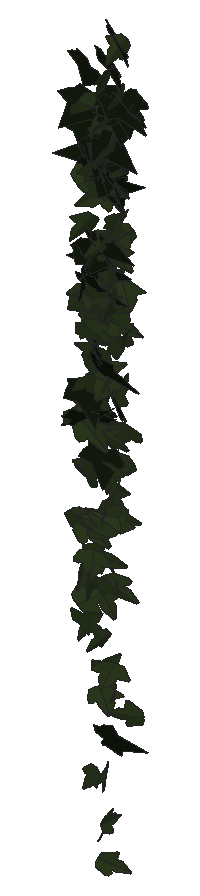
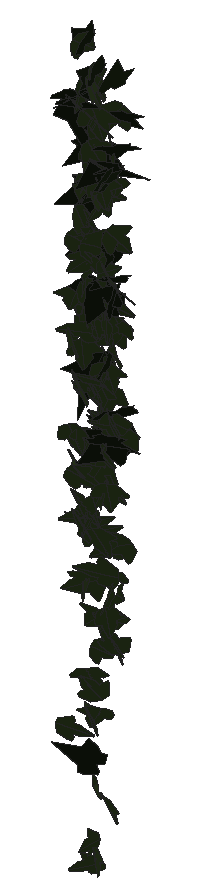
# SketchUp Ruby script. Lengths in inches.
U = 1.inch
M = Sketchup.active_model
def pt(a) = Geom::Point3d.new(a.map { |v| v * U })
def face(e, loops, mat)
  f = e.add_face(loops[0].map { |a| pt(a) })
  loops[1..].each { |l| e.add_face(l.map { |a| pt(a) }).erase! }
  f.material = f.back_material = mat if mat
  f
end
# faces: each face lists its corners as indices into pts; further lists are holes
def faces(e, pts, list, mat = nil) = list.each { |f| face(e, (f[0].is_a?(Array) ? f : [f]).map { |l| l.map { |i| pts[i] } }, mat) }
# xy, xz, yz: faces in a plane at the given z, y or x. An outline is a flat list of corners, or four numbers for a rectangle; further outlines are holes
def ring(l) = l.size == 4 ? [[l[0], l[1]], [l[2], l[1]], [l[2], l[3]], [l[0], l[3]]] : l.each_slice(2).to_a
def flat(e, list, mat, &to3) = list.each { |f| face(e, (f[0].is_a?(Array) ? f : [f]).map { |l| ring(l).map { |u, v| to3.(u, v) } }, mat) }
def xy(e, z, list, mat = nil) = flat(e, list, mat) { |x, y| [x, y, z] }
def xz(e, y, list, mat = nil) = flat(e, list, mat) { |x, z| [x, y, z] }
def yz(e, x, list, mat = nil) = flat(e, list, mat) { |y, z| [x, y, z] }
def lines(e, pts, list) = list.each { |a, b| e.add_line(pt(pts[a]), pt(pts[b])) }
# prism: a flat outline (further loops are holes) pulled along v
def prism(e, loops, v, mat = nil)
  f = face(e, loops, mat); d = Geom::Vector3d.new(v.map { |x| x * U })
  f.pushpull(f.normal.samedirection?(d) ? d.length : -d.length)
end
def box(e, o, s, mat = nil) = prism(e, [[o, [o[0] + s[0], o[1], o[2]], [o[0] + s[0], o[1] + s[1], o[2]], [o[0], o[1] + s[1], o[2]]]], [0, 0, s[2]], mat)
def at(x, y, z, deg = 0) = Geom::Transformation.translation(pt([x, y, z])) * Geom::Transformation.rotation(ORIGIN, Z_AXIS, deg.degrees)
def axes(o, x, y, z) = Geom::Transformation.new([*x, 0, *y, 0, *z, 0, *pt(o).to_a, 1])
def part(name) = M.definitions.add(name)
# library, detail: a bought-in or finely detailed component or shape, given as its bounding box
def library(name, o, s) = part(name).tap { |d| box(d.entities, o, s) }
def detail(e, o, s) = box(e.add_group.entities, o, s)
def put(e, d, t, mat = nil) = e.add_instance(d, t).tap { |i| i.material = mat if mat }
def group(e, t, mat = nil) = e.add_group.tap { |g| g.transformation = t; g.material = mat if mat }.entities
root = M.entities
M.materials.add("1026 AP 7946 SUNNY SIDE UP").color = [254, 231, 186]
M.materials.add("efeu1").color = [18, 25, 13]
M.materials.add("efeu2").color = [43, 57, 29]
c1 = part("ivyleaf_9")
p = [[1.54,2.16,1.25],[1.36,2.04,1.19],[-0.21,0.99,0.68],[-0.71,1.11,0.82],[-0.85,0.86,0.67],[-0.8,0.17,0.21],
  [-0.9,-0.01,0.1],[-0.67,-0.16,-0.02],[-0.08,-0.08,-0.05],[-0.03,-0.6,-0.4],[0.65,-0.88,-0.66],[0.83,-0.6,-0.49],
  [1.29,-0.42,-0.43],[1.8125,-0.07,-0.26],[1.21,0.44,0.15]]
faces(c1.entities,p,[[0,1,2,3,4,5,6,7,8,9,10,11,12,13,14]],"efeu1")
c2 = part("ivyleaf_10")
p = [[0,0.5,-0.03],[-0.0625,2.02,-0.43],[-0.19,2.01,-0.46],[-0.54,1.05,-0.29],[-0.52,0.625,-0.18],[-0.83,0.76,-0.28],
  [-1.16,0.64,-0.33],[-1.15,0.33,-0.24],[-0.77,-0.39,0.02],[-0.3,-0.51,0.16],[0.04,-0.48,0.23],[-0.02,2.01,-0.4375],
  [-0.06,2.01,-0.43],[0.04,-0.49,0.23],[0.67,-0.49,0.14],[1.38,0.36,-0.2],[1.375,0.51,-0.24],[0.81,0.65,-0.19],
  [0.62,0.59,-0.15],[0.6,1.09,-0.28],[0.5,1.23,-0.31]]
faces(c2.entities,p,[[0,1,2,3,4,5,6,7,8,9,10],[11,12,0,13,14,15,16,17,18,19,20]],"efeu2")
put(root,c1,axes([107.27,212.65,259.01],[-0.35146,-0.07913,0.09718],[-0.12704,-0.05448,-0.24347],[0.1468,-0.23659,0.02195]),"1026 AP 7946 SUNNY SIDE UP")
put(root,c1,axes([107.18,212.35,266.29],[-0.33681,-0.14799,0.05374],[-0.04557,-0.05088,-0.26728],[0.24294,-0.21471,0.02438]),"1026 AP 7946 SUNNY SIDE UP")
put(root,c1,axes([107.03,212.51,265.68],[-0.19517,-0.2139,-0.02355],[0.05901,0.00306,-0.25277],[0.33286,-0.12596,0.031]),"1026 AP 7946 SUNNY SIDE UP")
put(root,c2,axes([107.17,212.33,263.53],[-0.07974,-0.19065,0.17247],[-0.03607,-0.16768,-0.20355],[0.39844,-0.05333,0.01609]),"1026 AP 7946 SUNNY SIDE UP")
put(root,c2,axes([107.17,212.68,262.86],[-0.03382,0.04301,-0.23821],[-0.13272,-0.2184,-0.03501],[-0.34559,0.07966,0.03676]),"1026 AP 7946 SUNNY SIDE UP")
put(root,c2,axes([106.9,212.28,256.57],[-0.2205,0.00735,-0.19781],[0.29524,-0.04555,-0.14329],[-0.06456,-0.2334,0.02032]),"1026 AP 7946 SUNNY SIDE UP")
put(root,c2,axes([107.09,212.28,255.36],[0.01346,0.14801,-0.16409],[-0.02486,-0.1594,-0.1536],[-0.34197,0.01742,0.00471]),"1026 AP 7946 SUNNY SIDE UP")
put(root,c1,axes([107.03,212.5,262.22],[-0.00857,-0.00687,-0.25296],[0.26934,-0.17609,0.00013],[-0.27675,-0.17116,0.00796]),"1026 AP 7946 SUNNY SIDE UP")
put(root,c1,axes([107.41,212.5,265.09],[-0.31889,-0.00412,0.17125],[-0.25545,-0.05117,-0.20576],[0.05592,-0.2572,0.03663]),"1026 AP 7946 SUNNY SIDE UP")
put(root,c2,axes([106.97,212.62,259.47],[0.2066,-0.10808,0.16355],[0.19545,-0.09976,-0.17585],[0.23126,0.18086,0.00251]),"1026 AP 7946 SUNNY SIDE UP")
put(root,c2,axes([107.2,212.46,257.8],[-0.29258,-0.10467,0.03754],[-0.03402,-0.03671,-0.21908],[0.17124,-0.18614,0.02062]),"1026 AP 7946 SUNNY SIDE UP")
put(root,c2,axes([106.98,212.2,259.04],[-0.24658,-0.10244,-0.17997],[0.2466,0.0772,-0.19185],[0.20022,-0.22124,0.01466]),"1026 AP 7946 SUNNY SIDE UP")
put(root,c2,axes([107.17,212.33,261.53],[-0.23648,-0.16806,-0.00341],[0.02047,-0.00849,-0.23185],[0.26349,-0.15018,0.01495]),"1026 AP 7946 SUNNY SIDE UP")
put(root,c2,axes([107.17,212.51,255],[-0.13843,-0.20505,0.00708],[0.01022,-0.01152,-0.2297],[0.32251,-0.08765,0.01032]),"1026 AP 7946 SUNNY SIDE UP")
put(root,c2,axes([107.37,212.35,261.97],[-0.14813,-0.02247,0.22162],[-0.25618,-0.14717,-0.09015],[0.22401,-0.18317,0.04346]),"1026 AP 7946 SUNNY SIDE UP")
put(root,c1,axes([107.42,212.48,262.67],[-0.26739,0.15562,0.09575],[-0.13906,0.03865,-0.23536],[-0.24798,-0.18947,0.02874]),"1026 AP 7946 SUNNY SIDE UP")
put(root,c2,axes([107.02,212.32,261.58],[-0.28592,-0.06176,-0.12207],[0.20805,-0.0592,-0.17826],[0.02561,-0.20861,0.0853]),"1026 AP 7946 SUNNY SIDE UP")
put(root,c2,axes([107.4,212.18,257.7],[-0.02531,0.0288,0.2378],[-0.34752,0.06974,-0.02445],[-0.11325,-0.22045,0.02189]),"1026 AP 7946 SUNNY SIDE UP")
put(root,c2,axes([106.95,212.48,260.95],[0.12561,-0.03553,0.21534],[0.27654,-0.11404,-0.08979],[0.18677,0.19275,-0.01187]),"1026 AP 7946 SUNNY SIDE UP")
put(root,c1,axes([106.93,212.15,258.87],[0.24358,0.16582,-0.08438],[0.04295,0.08636,0.23121],[0.28828,-0.15297,0.03684]),"1026 AP 7946 SUNNY SIDE UP")
put(root,c2,axes([107.1875,212.48,261.71],[0.01596,-0.22356,-0.06441],[0.01796,0.06172,-0.22976],[0.36404,0.00675,0.01416]),"1026 AP 7946 SUNNY SIDE UP")
put(root,c2,axes([107.29,212.41,260.49],[-0.31761,-0.05874,0.07705],[-0.09814,-0.05161,-0.21476],[0.11338,-0.20924,0.02994]),"1026 AP 7946 SUNNY SIDE UP")
put(root,c1,axes([107.07,212.375,259.57],[-0.0634,-0.24999,-0.08098],[0.0215,0.07598,-0.26042],[0.41083,-0.04255,0.00113]),"1026 AP 7946 SUNNY SIDE UP")
put(root,c1,axes([107,212.5625,262.72],[0.03438,-0.21108,-0.12315],[0.07119,0.12029,-0.21172],[0.37379,-0.00349,0.05165]),"1026 AP 7946 SUNNY SIDE UP")
put(root,c2,axes([107.26,212.52,261.58],[-0.15796,-0.16653,0.15001],[-0.02283,-0.1556,-0.19331],[0.34807,-0.08578,0.0554]),"1026 AP 7946 SUNNY SIDE UP")
put(root,c2,axes([107.41,212.47,258.61],[0.02727,-0.04688,-0.22961],[-0.25417,0.15457,-0.0456],[0.25172,0.16115,-0.02117]),"1026 AP 7946 SUNNY SIDE UP")
put(root,c2,axes([107.2,212.24,254.21],[0.23113,-0.16519,0.00378],[-0.0126,-0.01329,-0.22737],[0.25955,0.14646,-0.01441]),"1026 AP 7946 SUNNY SIDE UP")
put(root,c2,axes([106.93,212.38,259.3],[0.17451,0.00598,-0.2306],[0.34215,0.05624,0.113],[0.08332,-0.24346,0.01894]),"1026 AP 7946 SUNNY SIDE UP")
put(root,c1,axes([107.11,212.43,267.02],[-0.12747,-0.16973,0.22097],[0.05951,-0.22944,-0.17288],[0.42715,-0.01868,0.09002]),"1026 AP 7946 SUNNY SIDE UP")
put(root,c2,axes([107.28,212.6,264.8],[-0.17533,-0.21789,0.03418],[-0.00679,-0.0364,-0.25203],[0.3468,-0.11087,0.01234]),"1026 AP 7946 SUNNY SIDE UP")
put(root,c2,axes([107.27,212.37,250.64],[0.24317,-0.14595,-0.03879],[-0.05607,0.01578,-0.21858],[0.22995,0.15819,-0.01227]),"1026 AP 7946 SUNNY SIDE UP")
put(root,c2,axes([107.11,212.26,254.15],[-0.27249,-0.04333,0.12948],[0.18418,0.04877,0.18362],[-0.09967,0.2086,-0.01469]),"1026 AP 7946 SUNNY SIDE UP")
put(root,c2,axes([107.24,212.48,262.9375],[0.17205,-0.24274,0.06822],[0.01884,-0.0686,-0.27416],[0.39576,0.1088,-0.01661]),"1026 AP 7946 SUNNY SIDE UP")
put(root,c1,axes([107.07,212.375,258.85],[0.34957,0.09701,0.06558],[0.10388,0.00581,-0.24896],[-0.1494,0.23102,-0.01968]),"1026 AP 7946 SUNNY SIDE UP")
put(root,c2,axes([107.15,212.17,266.31],[-0.16406,-0.14583,-0.22076],[0.22089,0.16126,-0.18328],[0.34124,-0.1745,0.01251]),"1026 AP 7946 SUNNY SIDE UP")
put(root,c1,axes([107.12,212.71,264.95],[0.05226,-0.20326,0.1472],[0.0136,-0.14429,-0.21265],[0.39148,0.03215,-0.01226]),"1026 AP 7946 SUNNY SIDE UP")
put(root,c2,axes([107.25,212.27,259.89],[-0.1655,-0.20571,-0.12208],[0.11652,0.09334,-0.23653],[0.35368,-0.12701,0.0208]),"1026 AP 7946 SUNNY SIDE UP")
put(root,c2,axes([107.36,212.16,260.39],[-0.01595,0.04964,0.25947],[-0.15963,0.23043,-0.04971],[-0.37027,-0.10148,0.01025]),"1026 AP 7946 SUNNY SIDE UP")
put(root,c1,axes([107.16,212.6,264.88],[-0.07846,-0.17988,0.17531],[0.06463,-0.17819,-0.18158],[0.38508,-0.00674,0.0662]),"1026 AP 7946 SUNNY SIDE UP")
put(root,c2,axes([107.12,212.2,254.6875],[0.18937,0.03532,-0.19977],[0.23407,0.133,0.12085],[0.20362,-0.18574,0.04686]),"1026 AP 7946 SUNNY SIDE UP")
put(root,c2,axes([107.04,212.55,259.37],[0.13889,0.00108,0.21341],[0.32564,-0.00545,-0.09098],[0.00722,0.22513,-0.00191]),"1026 AP 7946 SUNNY SIDE UP")
put(root,c2,axes([107.18,212.33,265.4],[-0.02226,0.04386,-0.26264],[0.11906,-0.2437,-0.04891],[-0.38936,-0.07703,0.00006]),"1026 AP 7946 SUNNY SIDE UP")
put(root,c1,axes([107.28,212.33,265.1875],[-0.01754,0.02952,-0.30196],[-0.14028,0.27939,0.0341],[0.44175,0.08989,-0.00116]),"1026 AP 7946 SUNNY SIDE UP")
put(root,c2,axes([107.33,212.64,264.6],[0.06378,-0.2093,0.11974],[0.01986,-0.11706,-0.22014],[0.37684,0.0416,-0.00866]),"1026 AP 7946 SUNNY SIDE UP")
put(root,c2,axes([107.37,212.11,255.22],[0.04121,-0.10601,-0.2445],[0.02175,0.23817,-0.1069],[0.40727,-0.002,0.03045]),"1026 AP 7946 SUNNY SIDE UP")
put(root,c2,axes([107.45,212.55,266.27],[-0.32454,-0.1257,0.07048],[-0.0637,-0.06513,-0.24698],[0.2164,-0.20769,0.03301]),"1026 AP 7946 SUNNY SIDE UP")
put(root,c2,axes([107.49,212.44,262.03],[-0.28562,0.08917,0.10765],[-0.17145,0.01042,-0.20536],[-0.13038,-0.20904,0.03423]),"1026 AP 7946 SUNNY SIDE UP")
put(root,c2,axes([107.4,212.25,264.9],[-0.07921,-0.25029,0.02683],[-0.00115,-0.02786,-0.26314],[0.39592,-0.05016,0.0046]),"1026 AP 7946 SUNNY SIDE UP")
put(root,c2,axes([107.52,212.44,256.65],[-0.28147,-0.05873,0.11833],[-0.15363,-0.06743,-0.19222],[0.13318,-0.20191,0.02836]),"1026 AP 7946 SUNNY SIDE UP")
put(root,c1,axes([107.15,212.4,263.18],[0.27025,-0.19402,0.00815],[-0.00976,-0.01752,-0.2666],[0.30526,0.17121,-0.01574]),"1026 AP 7946 SUNNY SIDE UP")
put(root,c2,axes([107.19,212.14,264.53],[0.1908,0.06517,-0.23116],[0.23299,0.17456,0.13558],[0.28481,-0.18647,0.04395]),"1026 AP 7946 SUNNY SIDE UP")
put(root,c2,axes([107.43,212.66,265.6],[-0.13892,-0.2061,0.10543],[-0.02164,-0.10594,-0.23002],[0.36201,-0.08543,0.02671]),"1026 AP 7946 SUNNY SIDE UP")
put(root,c2,axes([107.32,212.29,258.89],[-0.10809,0.20697,-0.09447],[0.03483,-0.09046,-0.22509],[-0.355,-0.07189,0.00668]),"1026 AP 7946 SUNNY SIDE UP")
put(root,c2,axes([107.15,212.24,256.38],[0.16936,0.10899,0.18382],[0.2284,0.10441,-0.15596],[-0.23533,0.17978,-0.01907]),"1026 AP 7946 SUNNY SIDE UP")
put(root,c2,axes([107.32,212.4,264.29],[-0.01192,-0.16702,-0.20093],[0.13893,0.18055,-0.16256],[0.37791,-0.07164,0.05342]),"1026 AP 7946 SUNNY SIDE UP")
put(root,c2,axes([107.31,212.24,255.77],[0.34273,0.05747,0.01362],[0.02812,-0.01748,-0.23127],[-0.08825,0.21765,-0.0208]),"1026 AP 7946 SUNNY SIDE UP")
put(root,c1,axes([107.36,212.4375,262.32],[0.29756,0.17356,-0.04665],[-0.03678,-0.04283,-0.2643],[-0.28004,0.19005,-0.01486]),"1026 AP 7946 SUNNY SIDE UP")
put(root,c2,axes([107.36,212.49,257.67],[-0.20351,0.15796,-0.06452],[0.04287,-0.05954,-0.21009],[-0.26425,-0.13131,0.01561]),"1026 AP 7946 SUNNY SIDE UP")
put(root,c1,axes([107.27,212.51,260.51],[0.00841,-0.12603,0.22475],[0.01649,-0.21863,-0.13123],[0.3968,0.01176,0.00069]),"1026 AP 7946 SUNNY SIDE UP")
put(root,c2,axes([107.4,212.45,261.42],[0.1389,-0.19141,0.11355],[-0.05421,0.10649,0.21746],[-0.34391,-0.09409,0.01158]),"1026 AP 7946 SUNNY SIDE UP")
put(root,c2,axes([107.49,212.46,249.43],[0.05444,-0.16766,-0.12683],[-0.05394,0.11752,-0.17548],[0.32169,0.04808,-0.00796]),"1026 AP 7946 SUNNY SIDE UP")
put(root,c2,axes([107.37,212.24,261.87],[0.13209,0.21012,0.07936],[0.03262,0.07333,-0.23256],[-0.34973,0.0862,0.00828]),"1026 AP 7946 SUNNY SIDE UP")
put(root,c2,axes([107.33,212.13,261.21],[-0.2739,-0.05275,-0.13983],[0.2116,0.02136,-0.18675],[0.08637,-0.21961,0.01406]),"1026 AP 7946 SUNNY SIDE UP")
put(root,c1,axes([107.14,212.32,261.98],[0.20909,-0.06903,0.21165],[0.25418,-0.12966,-0.15313],[0.22789,0.20795,-0.0234]),"1026 AP 7946 SUNNY SIDE UP")
put(root,c2,axes([107.53,212.44,259.95],[0.18685,-0.20218,-0.06677],[-0.06711,0.04866,-0.24101],[0.32647,0.12572,-0.01133]),"1026 AP 7946 SUNNY SIDE UP")
put(root,c2,axes([107.61,212.29,264.35],[0.11942,0.0958,-0.25708],[-0.25345,-0.19125,-0.12702],[-0.33631,0.17815,0.00444]),"1026 AP 7946 SUNNY SIDE UP")
put(root,c2,axes([107.5,212.6,266.98],[0.09253,-0.24822,0.06104],[0.01882,-0.0595,-0.26314],[0.40134,0.06002,-0.00173]),"1026 AP 7946 SUNNY SIDE UP")
put(root,c2,axes([107.25,212.16,258.79],[0.2495,0.0798,0.17169],[0.25272,0.04758,-0.18132],[-0.14205,0.22481,-0.02103]),"1026 AP 7946 SUNNY SIDE UP")
put(root,c2,axes([107.5,212.45,264.9375],[0.15188,-0.22277,0.03613],[0.01236,-0.03618,-0.25024],[0.35469,0.09665,-0.00675]),"1026 AP 7946 SUNNY SIDE UP")
put(root,c2,axes([107.48,212.52,266.01],[-0.02681,-0.08829,0.25464],[0.07674,-0.24495,-0.08792],[0.40627,0.04044,0.03341]),"1026 AP 7946 SUNNY SIDE UP")
put(root,c1,axes([107.3,212.65,264.62],[0.0941,-0.21633,0.11837],[0.06798,-0.10838,-0.23157],[0.38003,0.07295,0.01211]),"1026 AP 7946 SUNNY SIDE UP")
put(root,c2,axes([107.45,212.51,258.43],[-0.32948,0.0202,0.07866],[0.11392,-0.03626,0.21481],[0.04903,0.22001,0.02952]),"1026 AP 7946 SUNNY SIDE UP")
put(root,c2,axes([107.43,212.48,253.07],[-0.16577,-0.15189,0.11544],[0.07899,0.10217,0.19049],[-0.28693,0.11588,-0.01425]),"1026 AP 7946 SUNNY SIDE UP")
put(root,c2,axes([107.72,212.48,261.78],[-0.10181,-0.02067,0.22513],[-0.23723,-0.16147,-0.06269],[0.25097,-0.16102,0.03207]),"1026 AP 7946 SUNNY SIDE UP")
put(root,c2,axes([107.71,212.2,256.53],[0.11602,0.12255,0.18058],[-0.21073,-0.11708,0.14233],[0.26093,-0.14905,0.03466]),"1026 AP 7946 SUNNY SIDE UP")
put(root,c2,axes([107.59,212.3125,253.98],[-0.01451,-0.11878,0.1818],[-0.01001,-0.17708,-0.12369],[0.33521,-0.01043,0.00418]),"1026 AP 7946 SUNNY SIDE UP")
put(root,c1,axes([107.46,212.64,264.93],[-0.07289,-0.24051,0.00116],[0.00334,-0.00295,-0.25233],[0.37818,-0.04633,0.00245]),"1026 AP 7946 SUNNY SIDE UP")
put(root,c2,axes([107.59,212.38,267.08],[0.08511,-0.27022,0.03901],[-0.00068,-0.04025,-0.28402],[0.42939,0.0535,-0.00818]),"1026 AP 7946 SUNNY SIDE UP")
put(root,c2,axes([107.27,212.29,255.76],[0.00868,0.01198,0.26841],[0.36799,0.11465,-0.00987],[-0.18079,0.23394,-0.0072]),"1026 AP 7946 SUNNY SIDE UP")
put(root,c2,axes([107.68,212.42,263.18],[-0.03566,-0.11472,0.26018],[-0.05838,-0.25052,-0.12183],[0.43318,-0.04321,0.005]),"1026 AP 7946 SUNNY SIDE UP")
put(root,c2,axes([107.57,212.42,259.95],[0.39449,0.00865,-0.03697],[-0.05484,-0.02626,-0.2575],[-0.01924,0.25208,-0.02406]),"1026 AP 7946 SUNNY SIDE UP")
put(root,c2,axes([107.62,212.34,261.64],[-0.19944,-0.18709,-0.02541],[0.02953,0.01578,-0.23266],[0.29504,-0.12805,0.0061]),"1026 AP 7946 SUNNY SIDE UP")
put(root,c2,axes([107.64,212.59,262.3125],[-0.07694,-0.19644,0.1188],[-0.01203,-0.1176,-0.2084],[0.35887,-0.04606,0.01849]),"1026 AP 7946 SUNNY SIDE UP")
put(root,c2,axes([107.48,212.35,252.61],[0.23989,0.15316,0.0541],[0.07198,0.02716,-0.22215],[-0.24375,0.15876,-0.01236]),"1026 AP 7946 SUNNY SIDE UP")
put(root,c2,axes([107.59,212.55,252.625],[0.21863,-0.1994,0.03684],[0.01774,-0.03706,-0.25035],[0.31837,0.139,-0.01135]),"1026 AP 7946 SUNNY SIDE UP")
put(root,c2,axes([107.39,212.43,254.84],[0.28732,0.03383,0.14865],[0.22705,0.00963,-0.19089],[-0.05121,0.23251,-0.01234]),"1026 AP 7946 SUNNY SIDE UP")
put(root,c2,axes([107.61,212.35,249.59],[0.0268,-0.00697,0.2286],[-0.0705,0.2179,0.01188],[-0.34196,-0.04547,0.01547]),"1026 AP 7946 SUNNY SIDE UP")
put(root,c1,axes([107.39,212.62,267.23],[0.13887,-0.2222,0.11223],[0.05382,-0.10494,-0.24685],[0.38626,0.09451,-0.00595]),"1026 AP 7946 SUNNY SIDE UP")
put(root,c2,axes([107.39,212.38,260.13],[0.14813,-0.02701,-0.19746],[0.28545,0.08586,0.08002],[0.10495,-0.19541,0.06107]),"1026 AP 7946 SUNNY SIDE UP")
put(root,c1,axes([107.46,212.51,264.56],[0.13603,-0.22511,-0.03512],[-0.01437,0.03164,-0.24824],[0.35741,0.08695,0.00339]),"1026 AP 7946 SUNNY SIDE UP")
put(root,c2,axes([107.41,212.16,261.84],[-0.12032,-0.08076,0.20419],[0.25872,0.11317,0.11334],[-0.21626,0.18032,0.022]),"1026 AP 7946 SUNNY SIDE UP")
put(root,c2,axes([107.67,212.35,256.98],[-0.04539,0.10435,0.1883],[-0.10521,0.16975,-0.11008],[-0.31293,-0.07221,0.0097]),"1026 AP 7946 SUNNY SIDE UP")
put(root,c2,axes([107.55,212.37,256.99],[0.17583,-0.14623,0.13089],[0.12209,-0.10161,-0.19024],[0.28,0.13614,0.00076]),"1026 AP 7946 SUNNY SIDE UP")
put(root,c1,axes([107.55,212.57,264.88],[-0.07946,-0.22852,0.06871],[0.00847,-0.07058,-0.24066],[0.3748,-0.04685,0.02]),"1026 AP 7946 SUNNY SIDE UP")
put(root,c1,axes([107.42,212.15,263.22],[-0.00498,-0.0272,-0.26013],[0.18107,0.22475,-0.02513],[0.35566,-0.1148,0.00915]),"1026 AP 7946 SUNNY SIDE UP")
put(root,c2,axes([107.69,212.4,265.34],[-0.083,-0.22966,-0.09446],[0.03774,0.08721,-0.24222],[0.38624,-0.05787,0.00337]),"1026 AP 7946 SUNNY SIDE UP")
put(root,c1,axes([107.48,212.33,265.5],[-0.00101,-0.13442,-0.24977],[0.10417,0.23458,-0.13322],[0.4222,-0.0582,0.03227]),"1026 AP 7946 SUNNY SIDE UP")
put(root,c1,axes([107.95,212.43,266.29],[-0.23228,0.18031,0.10392],[-0.14092,0.05443,-0.23754],[-0.29184,-0.16979,0.03199]),"1026 AP 7946 SUNNY SIDE UP")
put(root,c1,axes([107.53,212.35,264.61],[0.17127,-0.21794,-0.10651],[-0.07227,0.09123,-0.25047],[0.3715,0.11822,0.00038]),"1026 AP 7946 SUNNY SIDE UP")
put(root,c2,axes([107.76,212.34,262.43],[-0.08096,0.1656,0.18919],[-0.13926,0.16178,-0.17581],[-0.36186,-0.0993,0.02533]),"1026 AP 7946 SUNNY SIDE UP")
put(root,c2,axes([107.91,212.61,257.98],[-0.14838,-0.03803,0.20541],[-0.24195,-0.13036,-0.10129],[0.20867,-0.17819,0.02862]),"1026 AP 7946 SUNNY SIDE UP")
put(root,c2,axes([107.64,212.15,258],[-0.38012,-0.02554,-0.08392],[0.13147,-0.02357,-0.24858],[0.02603,-0.25396,0.03]),"1026 AP 7946 SUNNY SIDE UP")
put(root,c2,axes([107.5,212.34,258.71],[-0.21368,-0.0052,-0.1957],[0.29813,-0.01901,-0.13933],[-0.01957,-0.23277,0.01438]),"1026 AP 7946 SUNNY SIDE UP")
put(root,c2,axes([107.7,212.375,258.83],[-0.31917,-0.09167,-0.05087],[0.08229,0.0024,-0.2286],[0.14109,-0.20876,0.01825]),"1026 AP 7946 SUNNY SIDE UP")
put(root,c1,axes([107.65,212.27,258.29],[-0.1483,-0.23097,-0.02272],[0.03027,0.01452,-0.25662],[0.36338,-0.09547,0.0121]),"1026 AP 7946 SUNNY SIDE UP")
put(root,c2,axes([107.42,212.32,264.5],[-0.00923,0.01048,0.26883],[0.41013,0.0122,0.00561],[-0.01882,0.26068,-0.00954]),"1026 AP 7946 SUNNY SIDE UP")
put(root,c2,axes([107.9,212.1875,256.65],[0.13697,0.13617,0.16461],[-0.20973,-0.09665,0.15997],[0.25372,-0.1534,0.04337]),"1026 AP 7946 SUNNY SIDE UP")
put(root,c2,axes([107.84,212.45,263.36],[0.142,0.14852,-0.16743],[-0.19373,-0.11257,-0.17625],[-0.28809,0.14891,0.03599]),"1026 AP 7946 SUNNY SIDE UP")
put(root,c2,axes([107.625,212.3,250.85],[0.11556,-0.06354,0.20672],[0.1944,-0.15945,-0.09942],[0.26851,0.14279,-0.01699]),"1026 AP 7946 SUNNY SIDE UP")
put(root,c1,axes([107.68,212.33,264.4],[-0.01977,0.11082,-0.2441],[-0.04808,0.2356,0.11626],[0.40939,0.03302,0.00186]),"1026 AP 7946 SUNNY SIDE UP")
put(root,c2,axes([107.55,212.6,257.27],[-0.13391,0.04195,0.21111],[0.31643,-0.04297,0.09508],[0.08835,0.21749,-0.02056]),"1026 AP 7946 SUNNY SIDE UP")
put(root,c2,axes([107.8125,212.49,260.88],[-0.22107,-0.18269,0.0075],[0.00968,-0.01521,-0.23713],[0.2874,-0.14001,0.01375]),"1026 AP 7946 SUNNY SIDE UP")
put(root,c2,axes([107.75,212.48,265.83],[0.24144,-0.19274,0.0505],[0.02718,-0.05015,-0.25353],[0.31196,0.15354,-0.017]),"1026 AP 7946 SUNNY SIDE UP")
put(root,c2,axes([107.76,212.63,264.63],[0.02563,-0.18615,0.16115],[0.05934,-0.15401,-0.19247],[0.37879,0.03673,0.01925]),"1026 AP 7946 SUNNY SIDE UP")
put(root,c1,axes([107.47,212.2,260.36],[0.35374,-0.0805,0.11987],[0.15759,-0.06483,-0.24524],[0.15789,0.24506,-0.0238]),"1026 AP 7946 SUNNY SIDE UP")
put(root,c2,axes([107.65,212.49,262.9],[-0.26404,-0.08807,-0.13648],[0.22548,-0.00197,-0.18661],[0.1068,-0.21357,0.05654]),"1026 AP 7946 SUNNY SIDE UP")
put(root,c2,axes([107.61,212.62,256.72],[0.13359,-0.11308,-0.19213],[0.19873,-0.13674,0.14443],[-0.27843,-0.15186,0.01091]),"1026 AP 7946 SUNNY SIDE UP")
put(root,c1,axes([107.89,212.4375,266.23],[0.25339,0.13151,-0.14656],[-0.19302,-0.07509,-0.21408],[-0.23679,0.20194,0.01768]),"1026 AP 7946 SUNNY SIDE UP")
put(root,c2,axes([107.83,212.25,253.33],[0.29265,0.09801,-0.07069],[-0.08538,-0.04502,-0.2165],[-0.1682,0.19339,-0.01309]),"1026 AP 7946 SUNNY SIDE UP")
put(root,c1,axes([107.51,212.48,251.48],[0.15979,-0.02789,0.22589],[0.29279,-0.11955,-0.10519],[0.18773,0.21019,-0.02821]),"1026 AP 7946 SUNNY SIDE UP")
put(root,c2,axes([107.92,212.61,263.36],[-0.11379,-0.08991,0.21697],[-0.05837,-0.21387,-0.10819],[0.35606,-0.06379,0.0516]),"1026 AP 7946 SUNNY SIDE UP")
put(root,c2,axes([107.86,212.54,267.78],[-0.08924,-0.12858,0.2233],[0.06257,-0.22467,-0.12745],[0.39231,0.00659,0.07112]),"1026 AP 7946 SUNNY SIDE UP")
put(root,c2,axes([108.08,212.28,261.69],[0.15675,-0.05607,-0.20919],[-0.25788,0.11978,-0.1165],[0.20713,0.19156,0.01327]),"1026 AP 7946 SUNNY SIDE UP")
put(root,c1,axes([107.67,212.59,267.85],[0.09805,-0.18424,0.18778],[0.05887,-0.18019,-0.20074],[0.40442,0.0709,-0.01631]),"1026 AP 7946 SUNNY SIDE UP")
put(root,c2,axes([107.92,212.42,263.8],[0.02208,-0.28885,0.05599],[0.00751,-0.05582,-0.29824],[0.46259,0.01469,0.00217]),"1026 AP 7946 SUNNY SIDE UP")
put(root,c2,axes([107.92,212.3,266.67],[-0.02056,-0.19102,-0.20015],[0.03721,0.19189,-0.19598],[0.42559,-0.02601,0.00747]),"1026 AP 7946 SUNNY SIDE UP")
put(root,c1,axes([107.74,212.53,264.5625],[0.05862,-0.2005,0.14415],[0.02103,-0.14081,-0.21065],[0.38491,0.03823,-0.01044]),"1026 AP 7946 SUNNY SIDE UP")
put(root,c2,axes([107.96,212.21,263.73],[0.25069,-0.20501,-0.0559],[-0.07268,0.03118,-0.26679],[0.32496,0.16512,-0.01654]),"1026 AP 7946 SUNNY SIDE UP")
put(root,c2,axes([107.64,212.47,261.24],[0.07225,0.04565,0.24142],[0.32558,0.11066,-0.06345],[-0.18609,0.21133,-0.01729]),"1026 AP 7946 SUNNY SIDE UP")
put(root,c2,axes([108.16,212.63,252.16],[-0.03864,-0.00038,0.22002],[-0.28087,-0.1178,-0.02208],[0.18408,-0.17983,0.0125]),"1026 AP 7946 SUNNY SIDE UP")
put(root,c2,axes([107.8,212.44,255.23],[-0.10507,0.05471,0.21348],[0.21227,-0.15743,0.08687],[0.26114,0.14998,0.01527]),"1026 AP 7946 SUNNY SIDE UP")
put(root,c1,axes([107.875,212.48,266.35],[-0.24828,-0.15822,-0.12152],[0.14205,0.07508,-0.22962],[0.27495,-0.18166,0.00889]),"1026 AP 7946 SUNNY SIDE UP")
put(root,c2,axes([107.86,212.29,256.7],[0.36768,-0.04466,-0.01452],[0.02808,0.02007,0.24421],[-0.06794,-0.23338,0.02236]),"1026 AP 7946 SUNNY SIDE UP")
put(root,c2,axes([108.09,212.5,258.86],[-0.293,-0.02645,0.10281],[-0.15148,-0.03036,-0.19349],[0.05902,-0.20926,0.01381]),"1026 AP 7946 SUNNY SIDE UP")
put(root,c2,axes([107.98,212.03,261.97],[0.01724,-0.19136,-0.21706],[0.01676,0.2099,-0.19561],[0.44597,-0.00049,0.01574]),"1026 AP 7946 SUNNY SIDE UP")
put(root,c2,axes([108.01,212.58,261.11],[0.04598,-0.21914,-0.00736],[-0.01112,0.005,-0.22764],[0.34452,0.02941,-0.00637]),"1026 AP 7946 SUNNY SIDE UP")
put(root,c2,axes([107.8,212.0625,248.9],[0.06589,0.08052,0.19825],[0.18199,0.15376,-0.09157],[-0.2721,0.12235,-0.01324]),"1026 AP 7946 SUNNY SIDE UP")
put(root,c2,axes([107.88,212.375,259.65],[0.26987,-0.20335,-0.03851],[0.05565,-0.01746,0.27356],[-0.31998,-0.17454,0.01509]),"1026 AP 7946 SUNNY SIDE UP")
put(root,c2,axes([107.79,212.22,256.86],[0.02395,0.03413,0.24266],[0.2188,0.18997,-0.03655],[-0.30324,0.13976,-0.00721]),"1026 AP 7946 SUNNY SIDE UP")
put(root,c1,axes([108.01,212.09,259.76],[0.25952,-0.05537,-0.18202],[-0.26565,0.05081,-0.179],[0.118,0.23615,-0.00265]),"1026 AP 7946 SUNNY SIDE UP")
put(root,c2,axes([107.92,212.53,262.1],[0.22085,0.18252,0.03764],[0.0347,0.02782,-0.23709],[-0.2903,0.14217,0.0003]),"1026 AP 7946 SUNNY SIDE UP")
put(root,c1,axes([107.91,212.51,266.62],[-0.15211,-0.24063,-0.10442],[0.07289,0.08907,-0.26649],[0.4032,-0.10688,0.00879]),"1026 AP 7946 SUNNY SIDE UP")
put(root,c2,axes([107.85,212.44,257.94],[0.05697,-0.1548,-0.15214],[0.17921,-0.11183,0.14981],[-0.28357,-0.10177,0.06411]),"1026 AP 7946 SUNNY SIDE UP")
put(root,c2,axes([107.82,212.2,255.375],[-0.24696,-0.04246,-0.20144],[0.31212,-0.00424,-0.16353],[0.03657,-0.25058,0.03539]),"1026 AP 7946 SUNNY SIDE UP")
put(root,c1,axes([107.82,212.32,266.57],[0.16056,-0.20782,-0.12911],[0.02796,0.14081,-0.22694],[0.37961,0.07752,0.07132]),"1026 AP 7946 SUNNY SIDE UP")
